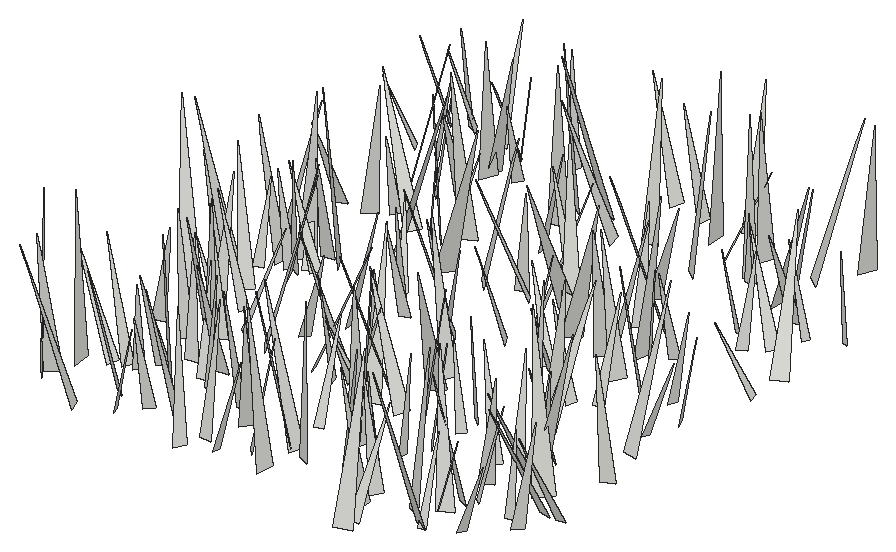
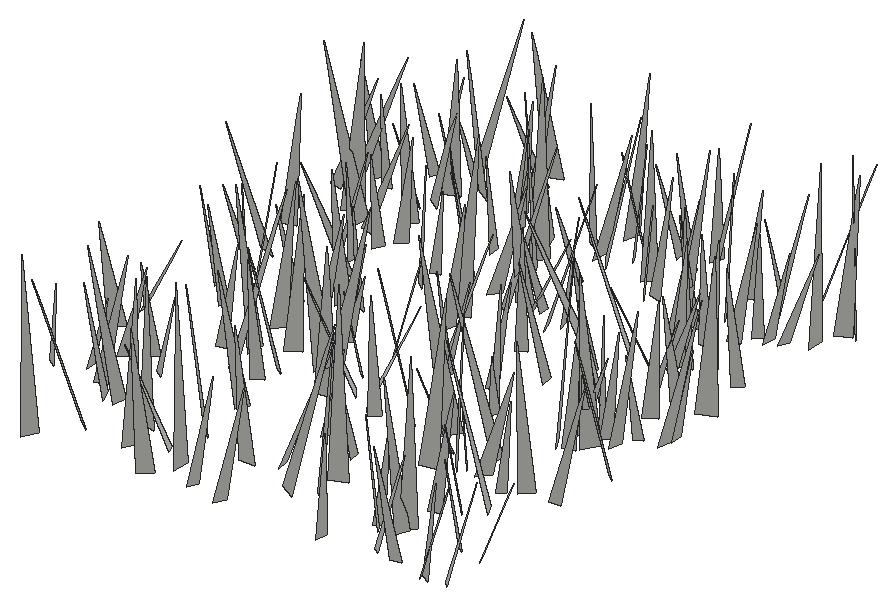
# SketchUp Ruby script. Lengths in inches.
U = 1.inch
M = Sketchup.active_model
def pt(a) = Geom::Point3d.new(a.map { |v| v * U })
def face(e, loops, mat)
  f = e.add_face(loops[0].map { |a| pt(a) })
  loops[1..].each { |l| e.add_face(l.map { |a| pt(a) }).erase! }
  f.material = f.back_material = mat if mat
  f
end
# faces: each face lists its corners as indices into pts; further lists are holes
def faces(e, pts, list, mat = nil) = list.each { |f| face(e, (f[0].is_a?(Array) ? f : [f]).map { |l| l.map { |i| pts[i] } }, mat) }
# xy, xz, yz: faces in a plane at the given z, y or x. An outline is a flat list of corners, or four numbers for a rectangle; further outlines are holes
def ring(l) = l.size == 4 ? [[l[0], l[1]], [l[2], l[1]], [l[2], l[3]], [l[0], l[3]]] : l.each_slice(2).to_a
def flat(e, list, mat, &to3) = list.each { |f| face(e, (f[0].is_a?(Array) ? f : [f]).map { |l| ring(l).map { |u, v| to3.(u, v) } }, mat) }
def xy(e, z, list, mat = nil) = flat(e, list, mat) { |x, y| [x, y, z] }
def xz(e, y, list, mat = nil) = flat(e, list, mat) { |x, z| [x, y, z] }
def yz(e, x, list, mat = nil) = flat(e, list, mat) { |y, z| [x, y, z] }
def lines(e, pts, list) = list.each { |a, b| e.add_line(pt(pts[a]), pt(pts[b])) }
# prism: a flat outline (further loops are holes) pulled along v
def prism(e, loops, v, mat = nil)
  f = face(e, loops, mat); d = Geom::Vector3d.new(v.map { |x| x * U })
  f.pushpull(f.normal.samedirection?(d) ? d.length : -d.length)
end
def box(e, o, s, mat = nil) = prism(e, [[o, [o[0] + s[0], o[1], o[2]], [o[0] + s[0], o[1] + s[1], o[2]], [o[0], o[1] + s[1], o[2]]]], [0, 0, s[2]], mat)
def at(x, y, z, deg = 0) = Geom::Transformation.translation(pt([x, y, z])) * Geom::Transformation.rotation(ORIGIN, Z_AXIS, deg.degrees)
def axes(o, x, y, z) = Geom::Transformation.new([*x, 0, *y, 0, *z, 0, *pt(o).to_a, 1])
def part(name) = M.definitions.add(name)
# library, detail: a bought-in or finely detailed component or shape, given as its bounding box
def library(name, o, s) = part(name).tap { |d| box(d.entities, o, s) }
def detail(e, o, s) = box(e.add_group.entities, o, s)
def put(e, d, t, mat = nil) = e.add_instance(d, t).tap { |i| i.material = mat if mat }
def group(e, t, mat = nil) = e.add_group.tap { |g| g.transformation = t; g.material = mat if mat }.entities
root = M.entities
c1 = part("fur_instance\#9")
p = [[0.8125,0,1.79],[0.67,-0.02,1.48],[0,-0.11,0],[0,0.11,0]]
faces(c1.entities,p,[[0,1,2,3]])
put(root,c1,axes([455.1,432.03,-21.66],[-7.08698,0.49693,1.41438],[0.58095,7.2106,0.37757],[1.38199,-0.48283,7.09434]))
put(root,c1,axes([454.9,430.87,-21.66],[-4.79431,0.50788,0.77321],[0.45097,4.84644,-0.38709],[0.80772,0.30866,4.80557]))
put(root,c1,axes([454.78,455.43,-21.66],[-3.14416,-1.79317,0.28571],[-1.75542,3.14785,0.43854],[0.46429,-0.24163,3.59289]))
put(root,c1,axes([454.56,460.0625,-21.66],[-3.11694,-3.18155,0.61605],[-3.14817,3.17551,0.47138],[0.76862,0.10457,4.42892]))
put(root,c1,axes([455.53,426.3,-21.66],[-4.19179,6.94453,1.88873],[7.18228,4.17546,0.58769],[0.45687,-1.92457,8.09026]))
put(root,c1,axes([454.47,408.96,-21.66],[-5.7343,-4.84539,3.53032],[-5.45543,6.24306,-0.29262],[2.4858,2.5238,7.50162]))
put(root,c1,axes([455.01,409.82,-21.66],[3.62749,-5.55241,1.8821],[-5.65778,-3.89547,-0.58748],[-1.5366,1.23544,6.60627]))
put(root,c1,axes([455.76,412.39,-21.66],[7.3985,0.06507,3.2704],[0.28828,-8.06925,-0.49163],[-3.25831,-0.56619,7.38244]))
put(root,c1,axes([455.9,444.78,-21.66],[1.11267,-4.69864,0.20362],[-4.67497,-1.12782,-0.47895],[-0.51316,0.0867,4.80478]))
put(root,c1,axes([456.39,460.4,-21.66],[-2.19445,-3.56039,1.55722],[-3.85398,2.22319,-0.34801],[0.4981,1.5159,4.16783]))
put(root,c1,axes([457.83,413.75,-21.66],[-4.93751,1.50851,0.32737],[1.53378,4.91815,0.47027],[0.1741,-0.54591,5.14135]))
put(root,c1,axes([456.87,460.37,-21.66],[-3.51503,-1.89548,0.64915],[-1.82323,3.56963,0.55065],[0.83071,-0.18586,3.95538]))
put(root,c1,axes([455.1875,438.77,-21.66],[3.97347,4.57155,1.31094],[4.73936,-3.94824,-0.59665],[-0.39506,-1.38509,6.02757]))
put(root,c1,axes([458,434.62,-21.66],[-6.22894,0.57755,1.75246],[0.68588,6.45268,0.31131],[1.71297,-0.48351,6.24791]))
put(root,c1,axes([459,414.14,-21.66],[-5.26641,1.25593,0.32091],[1.22212,5.2582,-0.5227],[0.43216,0.43524,5.3888]))
put(root,c1,axes([456.43,421.26,-21.66],[2.66304,-4.00114,1.09323],[-4.14622,-2.60379,0.57024],[-0.11461,1.22768,4.77239]))
put(root,c1,axes([457.17,432.74,-21.66],[-1.25475,3.57203,1.31412],[3.70812,1.4592,-0.42579],[0.858,-1.08261,3.76198]))
put(root,c1,axes([459.79,406.48,-21.66],[-6.57116,-2.81105,0.67584],[-2.85659,6.57143,-0.44162],[0.44572,0.67315,7.13352]))
put(root,c1,axes([458.62,429.44,-21.66],[3.00603,-4.02582,3.59921],[-4.80148,-3.87769,-0.32715],[-2.47129,2.63706,5.01362]))
put(root,c1,axes([457.17,455.07,-21.66],[2.36922,2.94645,1.17355],[3.15581,-2.33594,-0.5062],[-0.31572,-1.23846,3.7468]))
put(root,c1,axes([457.78,427.06,-21.66],[-1.16882,5.10436,1.64073],[5.31118,1.33199,-0.3603],[0.7334,-1.51127,5.22406]))
put(root,c1,axes([460.64,426.59,-21.66],[-4.9286,0.63717,0.02707],[0.62924,4.89286,-0.60144],[0.10377,0.59304,4.93308]))
put(root,c1,axes([459.24,434.125,-21.66],[-3.39336,2.50243,2.08506],[2.97495,3.60715,0.51243],[1.32637,-1.68843,4.18502]))
put(root,c1,axes([461.21,434.875,-21.66],[-4.19942,1.95994,0.17006],[1.96728,4.18576,0.33862],[0.01038,-0.37878,4.62189]))
put(root,c1,axes([458.67,444.86,-21.66],[3.92094,-4.8226,1.73149],[-5.06492,-3.97791,0.39007],[-0.77596,1.59628,6.20315]))
put(root,c1,axes([460.5,434.83,-21.66],[-2.92778,3.00983,0.00711],[2.98882,2.90849,-0.48849],[0.35507,0.33555,4.17041]))
put(root,c1,axes([459.98,420.26,-21.66],[1.65081,-5.08845,2.41171],[-5.51574,-1.96719,-0.37505],[-1.13372,2.16141,5.33637]))
put(root,c1,axes([459.32,436.04,-21.66],[6.01123,-4.10409,2.83515],[-4.50522,-6.3728,0.32708],[-2.14119,1.8869,7.27128]))
put(root,c1,axes([459.875,433.97,-21.66],[-2.18081,-4.36379,1.96245],[-4.63729,2.45895,0.31456],[1.17875,1.60022,4.86823]))
put(root,c1,axes([461.29,410.3,-21.66],[-3.14093,-4.54056,1.19879],[-4.68857,3.11384,-0.49041],[0.26658,1.26749,5.49924]))
put(root,c1,axes([459.9,459.68,-21.66],[-0.06431,5.36711,1.48252],[5.54585,0.19413,-0.46222],[0.49719,-1.47116,5.34755]))
put(root,c1,axes([460.3,446.03,-21.66],[2.53184,-2.74895,1.13947],[-2.76231,-2.72751,-0.44237],[-1.1067,0.51894,3.71097]))
put(root,c1,axes([460.02,414.26,-21.66],[3.44775,-2.42349,1.09947],[-2.43313,-3.5995,-0.30427],[-1.07797,0.37336,4.2033]))
put(root,c1,axes([462.99,444.77,-21.66],[-5.62336,3.63446,0.06059],[3.63174,5.6129,0.37548],[-0.15301,-0.3482,6.6851]))
put(root,c1,axes([462.16,422.3,-21.66],[-3.83694,1.86592,0.39498],[1.90547,3.78872,0.61201],[0.08273,-0.72368,4.22246]))
put(root,c1,axes([459.26,448.79,-21.66],[6.44327,3.68852,1.42181],[3.82977,-6.4983,-0.49739],[-0.97955,-1.14429,7.40767]))
put(root,c1,axes([460.53,437.22,-21.66],[1.15457,-5.41906,0.82486],[-5.48032,-1.12384,0.28761],[0.11275,0.86626,5.53322]))
put(root,c1,axes([460.95,450.17,-21.66],[3.02903,2.92229,1.12241],[2.89072,-3.2105,0.55771],[-1.2014,-0.35704,4.17178]))
put(root,c1,axes([461.09,415.91,-21.66],[1.69834,-4.62751,0.65795],[-4.61755,-1.76962,-0.52709],[-0.72459,0.43091,4.90106]))
put(root,c1,axes([460.12,432.88,-21.66],[5.04239,2.3615,1.06864],[2.46365,-5.09289,-0.37039],[-0.80566,-0.79378,5.55564]))
put(root,c1,axes([461.84,437.09,-21.66],[-6.4664,-4.252,2.80304],[-4.40658,6.94256,0.3657],[2.55316,1.21333,7.73047]))
put(root,c1,axes([462.0625,421.81,-21.66],[-4.31803,3.62073,2.04082],[3.93255,4.51165,0.31626],[1.34522,-1.56695,5.62628]))
put(root,c1,axes([462.17,459.29,-21.66],[-2.39227,-3.29447,0.41561],[-3.24315,2.42809,0.57931],[0.71291,-0.00928,4.03]))
put(root,c1,axes([461.58,421.31,-21.66],[-0.58668,-6.43534,2.37936],[-6.81319,0.82822,0.56013],[0.80964,2.30643,6.43771]))
put(root,c1,axes([462.41,417.83,-21.66],[-0.09344,5.23116,1.72248],[5.50098,0.0052,0.28262],[-0.26677,-1.725,5.22436]))
put(root,c1,axes([462.4,451.66,-21.66],[2.27929,-4.31761,0.37807],[-4.29346,-2.30768,-0.46977],[-0.59235,0.11282,4.85966]))
put(root,c1,axes([462.28,455.12,-21.66],[5.8288,-3.89293,1.62458],[-3.86791,-6.0381,-0.59132],[-1.68328,0.3943,6.98428]))
put(root,c1,axes([462.75,407.92,-21.66],[3.22488,1.438,0.95498],[1.40641,-3.36208,0.31327],[-1.00092,-0.09099,3.51704]))
put(root,c1,axes([464.18,413.05,-21.66],[-5.53367,-3.1899,2.46645],[-3.58117,5.81278,-0.51687],[1.85312,1.70777,6.3663]))
put(root,c1,axes([462.77,423.9,-21.66],[2.99625,3.60782,0.19235],[3.59342,-3.00177,0.328],[-0.37513,0.06212,4.67828]))
put(root,c1,axes([462.32,455.83,-21.66],[6.13982,-1.63324,0.91897],[-1.58888,-6.20592,-0.4139],[-0.99371,-0.16841,6.33984]))
put(root,c1,axes([464.97,416.03,-21.66],[-0.50295,4.78104,0.71911],[4.81704,0.43358,0.48636],[-0.41423,-0.76294,4.78276]))
put(root,c1,axes([464.6,409.89,-21.66],[2.46831,-3.73303,1.12427],[-3.72872,-2.64901,-0.60947],[-1.13849,0.58247,4.43358]))
put(root,c1,axes([464.51,418.42,-21.66],[-1.5232,-7.73744,1.34983],[-7.81047,1.63722,0.57115],[0.82858,1.20901,7.86523]))
put(root,c1,axes([464.49,456.05,-21.66],[2.8154,-3.04723,0.70248],[-2.99803,-2.89898,-0.55973],[-0.88933,0.126,4.11081]))
put(root,c1,axes([464.14,456.56,-21.66],[3.95435,2.54343,1.52337],[2.80761,-4.0284,-0.56212],[-0.95239,-1.31514,4.66797]))
put(root,c1,axes([464.8,444.6875,-21.66],[2.81827,1.89164,1.24112],[2.11841,-2.90244,-0.38665],[-0.79437,-1.02901,3.37216]))
put(root,c1,axes([465.52,417.83,-21.66],[0.67121,-5.58126,0.90748],[-5.6399,-0.72653,-0.2969],[-0.40679,0.86382,5.61363]))
put(root,c1,axes([465.55,445.05,-21.66],[4.83002,3.67653,3.08875],[4.26917,-5.29337,-0.3752],[-2.19806,-2.20219,6.05848]))
put(root,c1,axes([463.77,442.1,-21.66],[7.81228,1.65656,1.00866],[1.73052,-7.84393,-0.52089],[-0.87571,-0.72239,7.96898]))
put(root,c1,axes([466.83,460.3,-21.66],[-4.7956,1.01448,1.55419],[0.95492,5.04106,-0.34401],[1.59148,0.0322,4.88965]))
put(root,c1,axes([466.34,414.94,-21.66],[2.39277,4.07076,1.54907],[4.21231,-2.6123,0.35825],[-1.10775,-1.14055,4.7083]))
put(root,c1,axes([467.27,446.38,-21.66],[-2.10134,6.53759,3.4605],[7.38552,2.05442,0.60354],[0.41142,-3.48856,6.84043]))
put(root,c1,axes([465.71,422.94,-21.66],[6.07013,4.91373,1.22638],[4.90353,-6.18107,0.495],[-1.26656,-0.38061,7.79399]))
put(root,c1,axes([468.5,436.57,-21.66],[-2.98771,2.56269,0.00271],[2.54357,2.96592,-0.47684],[0.31249,0.36018,3.90722]))
put(root,c1,axes([467.53,443.21,-21.66],[2.30646,3.84948,0.31393],[3.83736,-2.32546,0.32205],[-0.43787,-0.10267,4.47599]))
put(root,c1,axes([466.91,426.44,-21.66],[3.70766,-2.56946,0.56874],[-2.62102,-3.69364,0.39947],[-0.23628,0.65362,4.49325]))
put(root,c1,axes([469.375,408,-21.66],[-6.2182,-2.45212,1.53392],[-2.39925,6.40419,0.51167],[1.61537,0.0727,6.66461]))
put(root,c1,axes([470.26,406.59,-21.66],[-5.1029,2.41175,1.4356],[2.37658,5.2976,-0.4521],[1.4931,-0.1897,5.62599]))
put(root,c1,axes([468.61,429.88,-21.66],[5.20805,0.62891,1.21236],[0.54515,-5.33937,0.42794],[-1.25226,0.29119,5.2284]))
put(root,c1,axes([470.33,414.25,-21.66],[-1.33118,-5.02308,1.66852],[-5.29255,1.28443,-0.35575],[0.06525,1.70478,5.18429]))
put(root,c1,axes([469.64,435.22,-21.66],[-0.67343,-4.75938,1.30258],[-4.88536,0.82798,0.49956],[0.69398,1.21023,4.78075]))
put(root,c1,axes([470.85,455.4,-21.66],[3.81307,5.29138,3.34018],[5.75803,-4.49829,0.55278],[-2.44962,-2.33704,6.49867]))
put(root,c1,axes([471.07,414.69,-21.66],[-3.53133,-2.30027,1.49102],[-2.55807,3.63918,-0.44418],[0.98523,1.20406,4.19097]))
put(root,c1,axes([471.09,433.68,-21.66],[0.8668,-4.44855,1.11397],[-4.54098,-0.99091,-0.42373],[-0.6404,1.00517,4.51236]))
put(root,c1,axes([471.12,408.67,-21.66],[0.82489,5.68831,1.342],[5.81529,-0.93413,0.38496],[-0.58339,-1.2684,5.73491]))
put(root,c1,axes([469.12,441.21,-21.66],[6.86151,-4.43995,0.81428],[-4.49635,-6.85344,0.51929],[-0.39875,0.87961,8.15621]))
put(root,c1,axes([473.5,456.27,-21.66],[-3.27464,-6.78559,1.40651],[-6.92909,3.22889,-0.5548],[0.10135,1.50857,7.51397]))
put(root,c1,axes([471.37,452.52,-21.66],[2.47243,-7.62212,2.09201],[-7.90302,-2.41845,0.52868],[-0.12434,2.1542,7.99563]))
put(root,c1,axes([474.02,423.25,-21.66],[-6.24569,-2.79636,0.92417],[-2.76847,6.31368,0.39421],[1.00464,0.01396,6.83176]))
put(root,c1,axes([470.65,422.91,-21.66],[5.67742,2.27779,0.25934],[2.25803,-5.67581,0.41845],[-0.39608,0.29237,6.10297]))
put(root,c1,axes([473.16,422.18,-21.66],[-4.36965,-1.59831,1.51111],[-1.58231,4.61869,0.30967],[1.52785,0.21216,4.64247]))
put(root,c1,axes([472.31,412.41,-21.66],[4.37125,-4.19897,0.80164],[-4.19734,-4.43318,-0.33332],[-0.81017,0.31203,6.05212]))
put(root,c1,axes([472.91,448.65,-21.66],[4.24313,0.45781,1.20359],[0.34307,-4.39664,0.46288],[-1.24117,0.34981,4.24258]))
put(root,c1,axes([472.875,407.83,-21.66],[4.10361,0.18993,0.89205],[0.09258,-4.17709,0.46346],[-0.90734,0.43277,4.08178]))
put(root,c1,axes([472.59,441.56,-21.66],[4.81614,4.80746,1.57054],[5.00941,-4.83285,-0.56818],[-0.69571,-1.51836,6.78115]))
put(root,c1,axes([473.18,427.39,-21.66],[1.74282,-4.6233,0.69197],[-4.67126,-1.6936,0.44965],[0.18179,0.80496,4.92038]))
put(root,c1,axes([475.42,433.84,-21.66],[-4.70558,-0.80345,0.83315],[-0.88013,4.74917,-0.39105],[0.7517,0.53106,4.75763]))
put(root,c1,axes([476.07,433.71,-21.66],[-5.08924,-4.37631,0.84531],[-4.44671,5.07308,-0.50754],[0.30556,0.93743,6.69289]))
put(root,c1,axes([476.3125,453.25,-21.66],[-6.23663,-1.3966,0.55844],[-1.37103,6.25805,0.33911],[0.61857,-0.21031,6.38209]))
put(root,c1,axes([476.96,441.92,-21.66],[-4.6266,-2.97065,0.07987],[-2.96143,4.59663,-0.58091],[-0.24706,0.53178,5.46742]))
put(root,c1,axes([476.55,421.88,-21.66],[-3.57731,-0.93265,0.01118],[-0.92223,3.54345,0.51048],[0.1395,-0.49118,3.66148]))
put(root,c1,axes([475.42,410.51,-21.66],[3.95748,1.9361,2.48086],[2.44941,-4.39763,-0.47534],[-1.97573,-1.57388,4.37997]))
put(root,c1,axes([476.62,460.83,-21.66],[-5.29366,2.0126,1.17564],[2.12712,5.36423,0.39489],[0.95291,-0.79376,5.64955]))
put(root,c1,axes([477.72,411.8,-21.66],[-6.93734,1.12272,0.61983],[1.08478,6.95591,-0.45824],[0.68406,0.3553,7.01265]))
put(root,c1,axes([476.79,412.3,-21.66],[-5.18557,-4.32883,1.54546],[-4.49087,5.26797,-0.31293],[0.97941,1.23577,6.74766]))
put(root,c1,axes([475.15,409.37,-21.66],[3.56693,3.32971,1.1246],[3.34181,-3.70943,0.38354],[-1.08812,-0.47732,4.86445]))
put(root,c1,axes([476.62,447.46,-21.66],[-3.90024,1.94852,0.94584],[2.05782,3.9414,0.36592],[0.67579,-0.75618,4.3445]))
put(root,c1,axes([475.125,433.85,-21.66],[4.21688,0.53755,0.91963],[0.65776,-4.26755,-0.52159],[-0.83787,-0.64478,4.21888]))
put(root,c1,axes([475.66,442.5625,-21.66],[2.40691,-4.24835,1.2679],[-4.42272,-2.4014,0.34948],[-0.30924,1.27831,4.87028]))
put(root,c1,axes([476.91,415.6875,-21.66],[0.03105,4.61747,0.04613],[4.59439,-0.03553,0.46309],[-0.46341,-0.04278,4.59429]))
put(root,c1,axes([475.76,421.32,-21.66],[4.29201,-0.29938,0.77765],[-0.39482,-4.32378,0.51456],[-0.73381,0.57535,4.27156]))
put(root,c1,axes([477.57,421.39,-21.66],[-1.40207,7.22786,1.13046],[7.31414,1.36087,0.37039],[-0.15287,-1.17973,7.35327]))
put(root,c1,axes([477.78,407.86,-21.66],[-7.15931,0.95304,2.49675],[1.12982,7.54938,0.35801],[2.42189,-0.70454,7.21359]))
put(root,c1,axes([478.25,423.17,-21.66],[-4.17901,-5.88434,0.7845],[-5.89024,4.22956,0.34775],[0.73891,0.43633,7.20893]))
put(root,c1,axes([479.9,428.21,-21.66],[-6.40273,2.01611,1.14645],[1.98655,6.50456,-0.34415],[1.19695,-0.01086,6.70383]))
put(root,c1,axes([478.82,454.6875,-21.66],[-0.28002,6.79198,1.74012],[7.00527,0.19856,0.35229],[-0.29175,-1.75129,6.78861]))
put(root,c1,axes([480.54,421.52,-21.66],[-5.38349,2.8617,0.60302],[2.91403,5.35589,0.59819],[0.24775,-0.81245,6.06741]))
put(root,c1,axes([479.19,410.9,-21.66],[3.04497,5.63186,2.55497],[5.93211,-3.46487,0.56775],[-1.7481,-1.94792,6.3771]))
put(root,c1,axes([479.85,460.11,-21.66],[-4.92159,1.07561,1.43405],[1.22896,5.07505,0.41117],[1.30503,-0.72281,5.02095]))
put(root,c1,axes([479.72,435.49,-21.66],[-3.92886,-2.51502,0.86647],[-2.44083,4.02285,0.60923],[1.05758,-0.05874,4.62495]))
put(root,c1,axes([479.08,440.73,-21.66],[4.55508,3.875,0.43107],[3.83788,-4.57312,0.55448],[-0.68713,0.14532,5.95457]))
put(root,c1,axes([481.54,441.42,-21.66],[-3.76745,6.43232,1.47995],[6.58457,3.78058,0.33053],[0.45645,-1.44608,7.44709]))
put(root,c1,axes([480.45,442.45,-21.66],[1.9178,-7.47283,0.23219],[-7.45531,-1.92947,-0.52008],[-0.56157,0.09505,7.69744]))
put(root,c1,axes([480.29,416.76,-21.66],[6.26613,3.81902,2.82967],[4.24719,-6.60086,-0.4964],[-2.13385,-1.92357,7.3214]))
put(root,c1,axes([480.49,438.2,-21.66],[2.6007,2.51832,0.88377],[2.64819,-2.58836,-0.41733],[-0.33183,-0.9193,3.59603]))
put(root,c1,axes([480.32,426.11,-21.66],[4.1786,-6.03386,0.40804],[-6.0035,-4.19846,-0.60465],[-0.72937,-0.01047,7.31455]))
put(root,c1,axes([481.125,415.1875,-21.66],[6.49174,-3.69034,2.54193],[-3.75607,-6.92147,-0.45599],[-2.44375,0.83512,7.45341]))
put(root,c1,axes([482.29,412.26,-21.66],[4.52412,1.43506,1.852],[1.32361,-4.8885,0.5546],[-1.93323,0.01133,4.71375]))
put(root,c1,axes([482.44,458.37,-21.66],[7.55648,0.00384,2.83421],[0.13477,-8.06186,-0.34839],[-2.831,-0.37353,7.54844]))
put(root,c1,axes([482.82,421.34,-21.66],[4.79862,3.05458,1.6678],[3.017,-5.06719,0.60002],[-1.73486,-0.36311,5.65661]))
put(root,c1,axes([484.73,434.62,-21.66],[-3.18645,2.79123,0.05753],[2.78151,3.16651,0.42911],[-0.23972,-0.36053,4.21429]))
put(root,c1,axes([484.01,460.875,-21.66],[-2.76968,5.79414,2.34049],[6.07448,3.09716,-0.47899],[1.46654,-1.88589,6.4042]))
put(root,c1,axes([485.49,412.12,-21.66],[-3.44021,1.49763,0.22694],[1.46636,3.43395,-0.43273],[0.37973,0.30751,3.72702]))
put(root,c1,axes([484.34,452.89,-21.66],[4.33311,5.30156,2.10924],[5.44411,-4.63436,0.46433],[-1.70794,-1.32191,6.83131]))
put(root,c1,axes([484.77,416.3,-21.66],[4.11345,0.18865,1.81103],[0.00918,-4.47631,0.44541],[-1.8208,0.4036,4.09361]))
put(root,c1,axes([485.76,411.67,-21.66],[-4.49863,-0.46507,1.40367],[-0.60193,4.68178,-0.37796],[1.35065,0.53749,4.50678]))
put(root,c1,axes([485.54,433.85,-21.66],[-1.12897,-3.54048,0.33773],[-3.515,1.16474,0.46018],[0.54205,0.17891,3.68752]))
put(root,c1,axes([486.12,421.94,-21.66],[1.74245,-3.02379,2.07472],[-3.3962,-2.19711,-0.34987],[-1.38332,1.58534,3.47232]))
put(root,c1,axes([483.3125,439.31,-21.66],[6.15872,-4.73604,0.69713],[-4.78091,-6.14284,0.50431],[-0.2428,0.82545,7.75278]))
put(root,c1,axes([485.84,424.21,-21.66],[-2.86919,-3.90872,1.79506],[-4.01549,3.2075,0.56601],[1.54149,1.08002,4.8156]))
put(root,c1,axes([485.67,418.82,-21.66],[3.79573,2.84609,1.46317],[3.05532,-3.89817,-0.34352],[-0.95191,-1.16307,4.73179]))
put(root,c1,axes([487.05,410.19,-21.66],[-4.02078,2.93374,1.78068],[3.22926,4.16274,0.43339],[1.1617,-1.41743,4.95839]))
put(root,c1,axes([484.59,447.97,-21.66],[4.6953,-3.04636,0.27903],[-3.0591,-4.67738,0.40996],[-0.01004,0.49581,5.58194]))
put(root,c1,axes([486.46,443.77,-21.66],[-2.20726,4.7722,2.01563],[5.04733,2.47451,-0.33147],[1.16667,-1.67676,5.24748]))
put(root,c1,axes([484.77,456.76,-21.66],[4.2362,2.18763,0.04516],[2.18011,-4.21144,-0.49393],[0.18673,-0.4595,4.74206]))
put(root,c1,axes([487.45,408.18,-21.66],[5.36084,-0.19835,3.29768],[0.06393,-6.27827,-0.48156],[-3.30302,-0.44345,5.34285]))
put(root,c1,axes([487.3125,429.95,-21.66],[1.36793,4.62634,1.5435],[4.80198,-1.5578,0.41343],[-0.85231,-1.35162,4.8066]))
put(root,c1,axes([486.0625,441.61,-21.66],[3.37327,4.28522,1.21914],[4.44713,-3.33099,-0.5966],[-0.2692,-1.33033,5.4209]))
put(root,c1,axes([487.1,438.5,-21.66],[3.86717,-5.0611,1.49434],[-5.13106,-4.03908,-0.40116],[-1.23289,0.93486,6.35679]))
put(root,c1,axes([488.72,444.26,-21.66],[-4.98525,-6.36904,1.05647],[-6.36247,5.07321,0.56124],[1.09531,0.48105,8.06861]))
put(root,c1,axes([487.59,458.22,-21.66],[6.10585,-2.9623,2.45846],[-2.96929,-6.55789,-0.52733],[-2.45002,0.56525,6.76598]))
put(root,c1,axes([488.53,455.05,-21.66],[1.00735,6.64791,2.58508],[7.07427,-1.26504,0.49655],[-0.91221,-2.46923,6.70544]))
put(root,c1,axes([488.4,404.29,-21.66],[-2.23719,7.0676,1.63885],[7.20712,2.3619,-0.34736],[0.83319,-1.45336,7.40509]))
put(root,c1,axes([488.31,405.75,-21.66],[-0.0626,5.05917,0.30688],[5.04763,0.09003,-0.45456],[0.45914,-0.29998,5.03909]))
put(root,c1,axes([489.94,430.94,-21.66],[-4.10178,1.61092,0.95507],[1.70987,4.15942,0.32775],[0.76391,-0.66031,4.39457]))
put(root,c1,axes([488.74,454.6,-21.66],[-0.48959,-3.44443,1.08487],[-3.54488,0.6673,0.51889],[0.68909,0.98557,3.44014]))
put(root,c1,axes([488.66,430.32,-21.66],[3.55242,-4.27149,1.91187],[-4.60398,-3.6203,0.46613],[-0.83917,1.77997,5.53606]))
put(root,c1,axes([490.32,436.26,-21.66],[-5.43342,3.18473,2.47254],[3.60205,5.6984,0.57576],[1.81141,-1.77869,6.27161]))
put(root,c1,axes([489.57,440.1875,-21.66],[6.98669,-0.82296,2.45735],[-1.02769,-7.36659,0.45485],[-2.37901,0.76535,7.02027]))
put(root,c1,axes([491.29,419.73,-21.66],[-3.65531,3.57205,1.42816],[3.77376,3.712,0.37448],[0.74692,-1.27356,5.09712]))
put(root,c1,axes([491.04,409.875,-21.66],[3.25616,5.95918,2.11371],[6.15078,-3.5363,0.49462],[-1.46542,-1.60155,6.77272]))
put(root,c1,axes([492.88,408.45,-21.66],[-3.74984,-6.28849,1.24601],[-6.40364,3.74219,-0.38514],[0.30173,1.26879,7.3115]))
put(root,c1,axes([491.78,441.55,-21.66],[1.41164,-4.04262,0.99191],[-4.10193,-1.52908,-0.39425],[-0.70768,0.79907,4.26381]))
put(root,c1,axes([491.24,426.42,-21.66],[0.40052,6.46259,0.29319],[6.45769,-0.38185,-0.40475],[0.38629,-0.31712,6.46233]))
put(root,c1,axes([492.99,411.41,-21.66],[-2.95923,6.17255,1.7602],[6.41346,2.92118,0.53848],[0.25723,-1.82266,6.82403]))
put(root,c1,axes([492.26,421.44,-21.66],[-3.32764,3.062,1.30373],[3.08153,3.53122,-0.42827],[1.25687,-0.55083,4.50173]))
put(root,c1,axes([491.84,431.96,-21.66],[-0.34341,4.80516,0.97397],[4.88667,0.41477,-0.32328],[0.39826,-0.94579,4.80656]))
put(root,c1,axes([493.12,413.38,-21.66],[-2.87551,-4.98025,1.4124],[-5.17006,2.84441,-0.49611],[0.26119,1.47404,5.72934]))
put(root,c1,axes([493.02,447.93,-21.66],[-1.62958,-3.15436,1.09529],[-3.33909,1.53504,-0.54711],[-0.01197,1.22427,3.50802]))
put(root,c1,axes([493.23,408.13,-21.66],[0.25291,3.93977,0.05992],[3.89833,-0.25892,0.57035],[-0.57304,-0.02262,3.90646]))
put(root,c1,axes([492.21,411.55,-21.66],[3.27913,1.40298,0.59687],[1.4938,-3.23974,-0.59158],[-0.30522,-0.78299,3.51725]))
put(root,c1,axes([492.57,424.36,-21.66],[3.92592,-0.41216,0.89749],[-0.2951,-4.00034,-0.54626],[-0.94248,-0.46433,3.90952]))
put(root,c1,axes([492.6,457.88,-21.66],[4.44163,5.80553,0.93246],[5.82565,-4.50337,0.28854],[-0.79717,-0.56325,7.30404]))
put(root,c1,axes([493.3,436.3125,-21.66],[-3.24328,-4.06122,2.56752],[-4.33534,3.80899,0.54855],[2.07134,1.61325,5.16831]))
put(root,c1,axes([492.73,416.84,-21.66],[3.51068,-4.45404,1.06123],[-4.56743,-3.50052,0.41776],[-0.32136,1.09429,5.65587]))
put(root,c1,axes([494.74,422.83,-21.66],[-2.89308,-3.13599,0.85003],[-3.23039,2.89836,-0.3018],[0.34876,0.83187,4.25597]))
put(root,c1,axes([494.59,420.01,-21.66],[-0.95692,-4.60949,0.0097],[-4.59629,0.95343,-0.35816],[-0.34872,0.08227,4.69412]))
put(root,c1,axes([494.96,433.68,-21.66],[-5.04486,-3.51647,1.75014],[-3.733,5.17856,-0.35556],[1.22196,1.30239,6.1392]))
put(root,c1,axes([493.96,414.22,-21.66],[2.60004,3.22909,0.64132],[3.22546,-2.66223,0.32783],[-0.65933,-0.2899,4.13277]))
put(root,c1,axes([494.07,453.3,-21.66],[4.8135,2.02359,1.54657],[1.94555,-5.05552,0.55956],[-1.64367,-0.05793,5.19149]))
put(root,c1,axes([492.67,453.32,-21.66],[6.50661,-0.43072,0.76621],[-0.39332,-6.54513,-0.33931],[-0.78607,-0.29036,6.51202]))
put(root,c1,axes([496.92,447.47,-21.66],[-4.22119,3.06488,0.48562],[3.10212,4.18863,0.52921],[0.07866,-0.71394,5.1896]))
put(root,c1,axes([495.02,445.96,-21.66],[2.53545,-3.02814,1.98338],[-3.53036,-2.60371,0.53779],[-0.80002,1.89288,3.91266]))
put(root,c1,axes([495.66,451.91,-21.66],[1.37303,-5.10418,0.31363],[-5.09334,-1.39399,-0.38851],[-0.45708,0.20095,5.27134]))
put(root,c1,axes([494.86,461.76,-21.66],[6.65936,-3.07974,1.86174],[-3.09449,-6.89952,-0.34452],[-1.83712,0.458,7.32893]))
put(root,c1,axes([497.51,418.05,-21.66],[-5.36752,5.77658,2.45123],[6.12108,5.53013,0.37117],[1.38195,-2.05828,7.87664]))
put(root,c1,axes([497.94,450.28,-21.66],[-4.0966,0.35691,0.30901],[0.31396,4.07547,-0.54495],[0.35257,0.51784,4.07585]))
put(root,c1,axes([496.09,435.97,-21.66],[4.13039,-0.87619,1.21239],[-0.99071,-4.26996,0.28929],[-1.12075,0.54542,4.21238]))
put(root,c1,axes([495.9375,409.71,-21.66],[3.40491,-1.73217,0.1961],[-1.74293,-3.39081,0.31125],[-0.03288,0.3664,3.80749]))
put(root,c1,axes([495.8,419.29,-21.66],[7.40162,-2.04644,1.37858],[-2.14984,-7.48787,0.42713],[-1.21103,0.78507,7.66743]))
put(root,c1,axes([497.63,413.62,-21.66],[0.95056,-3.70171,1.6828],[-4.06505,-0.90725,0.30052],[-0.09921,1.70654,3.80998]))
put(root,c1,axes([499.34,415.86,-21.66],[-1.38983,-5.84462,0.0201],[-5.82782,1.38425,-0.46046],[-0.44334,0.12603,5.98992]))
put(root,c1,axes([498.6,427.43,-21.66],[1.7832,7.11152,0.69499],[7.11724,-1.83129,0.47737],[-0.63379,-0.55606,7.31612]))
put(root,c1,axes([497.63,430.69,-21.66],[3.74369,-0.67268,0.40161],[-0.71907,-3.7286,0.45768],[-0.31101,0.52348,3.776]))
put(root,c1,axes([500.375,440.65,-21.66],[-3.53813,-0.73541,0.01575],[-0.72603,3.50386,0.50526],[0.11809,-0.49152,3.57826]))
put(root,c1,axes([500.32,443.99,-21.66],[-3.69849,5.78351,0.10997],[5.76561,3.69627,-0.48502],[0.46777,0.16892,6.84781]))
put(root,c1,axes([498.56,433.8,-21.66],[3.70099,1.78589,1.07617],[1.91017,-3.78303,-0.29128],[-0.83593,-0.7377,4.09901]))
put(root,c1,axes([500.03,422.96,-21.66],[1.93856,-5.12728,2.24723],[-5.46022,-2.25638,-0.43794],[-1.23493,1.9279,5.46399]))
put(root,c1,axes([499.18,412.73,-21.66],[4.20018,-2.603,1.54886],[-2.85846,-4.28223,0.55487],[-1.0019,1.30501,4.91012]))
put(root,c1,axes([500.65,451.72,-21.66],[1.66971,3.21733,1.57549],[3.35444,-2.01427,0.55833],[-1.25742,-1.10127,3.58153]))
put(root,c1,axes([500.91,415.875,-21.66],[-0.25255,-4.7231,0.0991],[-4.68784,0.23828,-0.59045],[-0.58449,0.12972,4.69284]))
